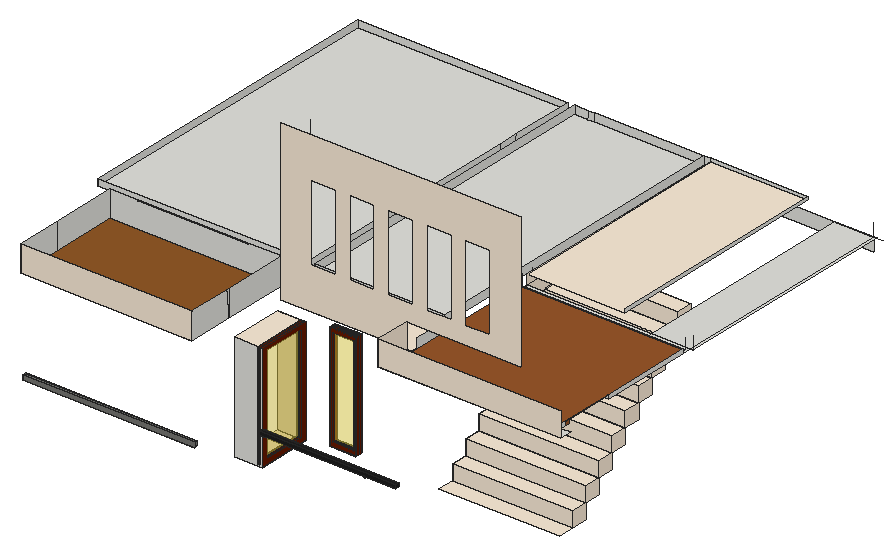
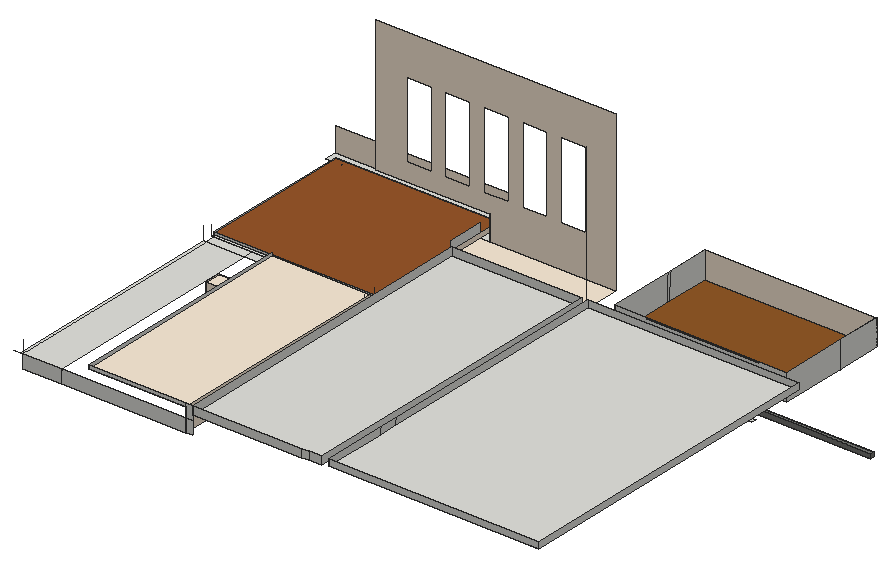
# SketchUp Ruby script. Lengths in inches.
U = 1.inch
M = Sketchup.active_model
def pt(a) = Geom::Point3d.new(a.map { |v| v * U })
def face(e, loops, mat)
  f = e.add_face(loops[0].map { |a| pt(a) })
  loops[1..].each { |l| e.add_face(l.map { |a| pt(a) }).erase! }
  f.material = f.back_material = mat if mat
  f
end
# faces: each face lists its corners as indices into pts; further lists are holes
def faces(e, pts, list, mat = nil) = list.each { |f| face(e, (f[0].is_a?(Array) ? f : [f]).map { |l| l.map { |i| pts[i] } }, mat) }
# xy, xz, yz: faces in a plane at the given z, y or x. An outline is a flat list of corners, or four numbers for a rectangle; further outlines are holes
def ring(l) = l.size == 4 ? [[l[0], l[1]], [l[2], l[1]], [l[2], l[3]], [l[0], l[3]]] : l.each_slice(2).to_a
def flat(e, list, mat, &to3) = list.each { |f| face(e, (f[0].is_a?(Array) ? f : [f]).map { |l| ring(l).map { |u, v| to3.(u, v) } }, mat) }
def xy(e, z, list, mat = nil) = flat(e, list, mat) { |x, y| [x, y, z] }
def xz(e, y, list, mat = nil) = flat(e, list, mat) { |x, z| [x, y, z] }
def yz(e, x, list, mat = nil) = flat(e, list, mat) { |y, z| [x, y, z] }
def lines(e, pts, list) = list.each { |a, b| e.add_line(pt(pts[a]), pt(pts[b])) }
# prism: a flat outline (further loops are holes) pulled along v
def prism(e, loops, v, mat = nil)
  f = face(e, loops, mat); d = Geom::Vector3d.new(v.map { |x| x * U })
  f.pushpull(f.normal.samedirection?(d) ? d.length : -d.length)
end
def box(e, o, s, mat = nil) = prism(e, [[o, [o[0] + s[0], o[1], o[2]], [o[0] + s[0], o[1] + s[1], o[2]], [o[0], o[1] + s[1], o[2]]]], [0, 0, s[2]], mat)
def at(x, y, z, deg = 0) = Geom::Transformation.translation(pt([x, y, z])) * Geom::Transformation.rotation(ORIGIN, Z_AXIS, deg.degrees)
def axes(o, x, y, z) = Geom::Transformation.new([*x, 0, *y, 0, *z, 0, *pt(o).to_a, 1])
def part(name) = M.definitions.add(name)
# library, detail: a bought-in or finely detailed component or shape, given as its bounding box
def library(name, o, s) = part(name).tap { |d| box(d.entities, o, s) }
def detail(e, o, s) = box(e.add_group.entities, o, s)
def put(e, d, t, mat = nil) = e.add_instance(d, t).tap { |i| i.material = mat if mat }
def group(e, t, mat = nil) = e.add_group.tap { |g| g.transformation = t; g.material = mat if mat }.entities
root = M.entities
M.materials.add("[0028_AntiqueWhite]").color = [250, 235, 215]
M.materials.add("[Color B08]").color = [102, 25, 0]
M.materials.add("[Color M00]").color = [255, 255, 255]
M.materials.add("[Color M08]").color = [30, 30, 30]
M.materials.add("[Metal Seamed]").color = [118, 119, 115]
M.materials.add("[Translucent Glass Blue]").color = [255, 231, 67]
M.materials["[Translucent Glass Blue]"].alpha = 0.5
M.materials.add("[Wood Cherry Original]").color = [152, 86, 42]
M.materials.add("[Wood Floor Parquet]").color = [145, 89, 39]
c1 = part("Group\#3")
xy(c1.entities,0,[[0,0,22,2.875],[0,2.875,22,5.5]],"[Color B08]")
xy(c1.entities,2.22,[[2.22,0,19.78,2.875],[2.22,2.875,19.78,5.5]],"[Color B08]")
xy(c1.entities,55.28,[[2.22,0,19.78,2.875],[2.22,2.875,19.78,5.5]],"[Color B08]")
xy(c1.entities,57.5,[[0,0,22,2.875],[0,2.875,22,5.5]],"[Color B08]")
xz(c1.entities,0,[[[0,0,22,57.5],[2.22,2.22,19.78,55.28]]],"[Color B08]")
xz(c1.entities,2.875,[[[0,0,22,57.5],[2.22,2.22,19.78,55.28]]],"[Color B08]")
xz(c1.entities,2.875,[[2.22,2.22,19.78,55.28]],"[Translucent Glass Blue]")
xz(c1.entities,5.5,[[[0,0,22,57.5],[2.22,2.22,19.78,55.28]]],"[Color B08]")
yz(c1.entities,0,[[0,0,2.875,57.5],[2.875,0,5.5,57.5]],"[Color B08]")
yz(c1.entities,2.22,[[0,2.22,2.875,55.28],[2.875,2.22,5.5,55.28]],"[Color B08]")
yz(c1.entities,19.78,[[0,2.22,2.875,55.28],[2.875,2.22,5.5,55.28]],"[Color B08]")
yz(c1.entities,22,[[0,0,2.875,57.5],[2.875,0,5.5,57.5]],"[Color B08]")
c2 = part("Group\#8")
box(c2.entities,[0,0,0],[51.12,12,8])
xy(root,181.1,[[206.5625,238.8,232.3125,288.24]],"[0028_AntiqueWhite]")
xy(root,181.75,[[249.93,292.4375,274.3,298.4375]])
xy(root,187.49,[[355.75,284.99,465.14,299.89]],"[0028_AntiqueWhite]")
xy(root,208.625,[[173.42,194.68,173.5625,194.68,173.71,194.72,173.83,194.79,173.9375,194.89,174.01,195.02,174.05,195.16,174.05,195.31,174.01,195.45,173.94,195.58,173.83,195.68,173.7,195.75,173.5625,195.79,173.42,195.79,173.27,195.75,173.15,195.68,173.04,195.58,172.97,195.45,172.93,195.31,172.93,195.16,172.97,195.02,173.04,194.89,173.15,194.79,173.28,194.71]],"[Color M08]")
xy(root,208.66,[[[50.75,193.58,206.5625,196.4375],[54.79,194.68,54.9375,194.68,55.08,194.72,55.21,194.79,55.3125,194.89,55.38,195.02,55.42,195.16,55.42,195.31,55.38,195.45,55.31,195.58,55.21,195.68,55.08,195.75,54.9375,195.79,54.79,195.79,54.65,195.75,54.52,195.68,54.42,195.58,54.34,195.45,54.31,195.31,54.31,195.16,54.35,195.02,54.42,194.89,54.52,194.79,54.65,194.71],[59.35,194.68,59.5,194.68,59.64,194.72,59.77,194.79,59.875,194.89,59.95,195.02,59.99,195.16,59.98,195.31,59.95,195.45,59.87,195.58,59.77,195.68,59.64,195.75,59.5,195.79,59.35,195.79,59.21,195.75,59.08,195.68,58.98,195.58,58.91,195.45,58.87,195.31,58.87,195.16,58.91,195.02,58.98,194.89,59.09,194.79,59.21,194.71],[63.92,194.68,64.0625,194.68,64.21,194.72,64.33,194.79,64.4375,194.89,64.51,195.02,64.55,195.16,64.55,195.31,64.51,195.45,64.44,195.58,64.33,195.68,64.2,195.75,64.0625,195.79,63.92,195.79,63.77,195.75,63.65,195.68,63.54,195.58,63.47,195.45,63.43,195.31,63.43,195.16,63.47,195.02,63.54,194.89,63.65,194.79,63.78,194.71],[68.48,194.68,68.625,194.68,68.77,194.72,68.9,194.79,69,194.89,69.07,195.02,69.11,195.16,69.11,195.31,69.07,195.45,69,195.58,68.89,195.68,68.77,195.75,68.625,195.79,68.48,195.79,68.34,195.75,68.21,195.68,68.11,195.58,68.03,195.45,67.99,195.31,67.99,195.16,68.03,195.02,68.11,194.89,68.21,194.79,68.34,194.71],[73.04,194.68,73.1875,194.68,73.33,194.72,73.46,194.79,73.5625,194.89,73.63,195.02,73.67,195.16,73.67,195.31,73.63,195.45,73.56,195.58,73.46,195.68,73.33,195.75,73.1875,195.79,73.04,195.79,72.9,195.75,72.77,195.68,72.67,195.58,72.59,195.45,72.56,195.31,72.56,195.16,72.6,195.02,72.67,194.89,72.77,194.79,72.9,194.71],[77.6,194.68,77.75,194.68,77.89,194.72,78.02,194.79,78.125,194.89,78.2,195.02,78.24,195.16,78.23,195.31,78.2,195.45,78.12,195.58,78.02,195.68,77.89,195.75,77.75,195.79,77.6,195.79,77.46,195.75,77.33,195.68,77.23,195.58,77.16,195.45,77.12,195.31,77.12,195.16,77.16,195.02,77.23,194.89,77.34,194.79,77.46,194.71],[82.17,194.68,82.3125,194.68,82.46,194.72,82.58,194.79,82.6875,194.89,82.76,195.02,82.8,195.16,82.8,195.31,82.76,195.45,82.69,195.58,82.58,195.68,82.45,195.75,82.3125,195.79,82.17,195.79,82.02,195.75,81.9,195.68,81.79,195.58,81.72,195.45,81.68,195.31,81.68,195.16,81.72,195.02,81.79,194.89,81.9,194.79,82.03,194.71],[86.73,194.68,86.875,194.68,87.02,194.72,87.15,194.79,87.25,194.89,87.32,195.02,87.36,195.16,87.36,195.31,87.32,195.45,87.25,195.58,87.14,195.68,87.02,195.75,86.875,195.79,86.73,195.79,86.59,195.75,86.46,195.68,86.36,195.58,86.28,195.45,86.24,195.31,86.24,195.16,86.28,195.02,86.36,194.89,86.46,194.79,86.59,194.71],[91.29,194.68,91.4375,194.68,91.58,194.72,91.71,194.79,91.8125,194.89,91.88,195.02,91.92,195.16,91.92,195.31,91.88,195.45,91.81,195.58,91.71,195.68,91.58,195.75,91.4375,195.79,91.29,195.79,91.15,195.75,91.02,195.68,90.92,195.58,90.84,195.45,90.81,195.31,90.81,195.16,90.85,195.02,90.92,194.89,91.02,194.79,91.15,194.71],[95.85,194.68,96,194.68,96.14,194.72,96.27,194.79,96.375,194.89,96.45,195.02,96.49,195.16,96.48,195.31,96.45,195.45,96.37,195.58,96.27,195.68,96.14,195.75,96,195.79,95.85,195.79,95.71,195.75,95.58,195.68,95.48,195.58,95.41,195.45,95.37,195.31,95.37,195.16,95.41,195.02,95.48,194.89,95.59,194.79,95.71,194.71],[104.98,194.68,105.125,194.68,105.27,194.72,105.4,194.79,105.5,194.89,105.57,195.02,105.61,195.16,105.61,195.31,105.57,195.45,105.5,195.58,105.39,195.68,105.27,195.75,105.125,195.79,104.98,195.79,104.84,195.75,104.71,195.68,104.61,195.58,104.53,195.45,104.49,195.31,104.49,195.16,104.53,195.02,104.61,194.89,104.71,194.79,104.84,194.71],[109.54,194.68,109.6875,194.68,109.83,194.72,109.96,194.79,110.0625,194.89,110.13,195.02,110.17,195.16,110.17,195.31,110.13,195.45,110.06,195.58,109.96,195.68,109.83,195.75,109.6875,195.79,109.54,195.79,109.4,195.75,109.27,195.68,109.17,195.58,109.09,195.45,109.06,195.31,109.06,195.16,109.1,195.02,109.17,194.89,109.27,194.79,109.4,194.71],[114.1,194.68,114.25,194.68,114.39,194.72,114.52,194.79,114.625,194.89,114.7,195.02,114.74,195.16,114.73,195.31,114.7,195.45,114.62,195.58,114.52,195.68,114.39,195.75,114.25,195.79,114.1,195.79,113.96,195.75,113.83,195.68,113.73,195.58,113.66,195.45,113.62,195.31,113.62,195.16,113.66,195.02,113.73,194.89,113.84,194.79,113.96,194.71],[118.67,194.68,118.8125,194.68,118.96,194.72,119.08,194.79,119.1875,194.89,119.26,195.02,119.3,195.16,119.3,195.31,119.26,195.45,119.19,195.58,119.08,195.68,118.95,195.75,118.8125,195.79,118.67,195.79,118.52,195.75,118.4,195.68,118.29,195.58,118.22,195.45,118.18,195.31,118.18,195.16,118.22,195.02,118.29,194.89,118.4,194.79,118.53,194.71],[123.23,194.68,123.375,194.68,123.52,194.72,123.65,194.79,123.75,194.89,123.82,195.02,123.86,195.16,123.86,195.31,123.82,195.45,123.75,195.58,123.64,195.68,123.52,195.75,123.375,195.79,123.23,195.79,123.09,195.75,122.96,195.68,122.86,195.58,122.78,195.45,122.74,195.31,122.74,195.16,122.78,195.02,122.86,194.89,122.96,194.79,123.09,194.71],[127.79,194.68,127.9375,194.68,128.08,194.72,128.21,194.79,128.3125,194.89,128.38,195.02,128.42,195.16,128.42,195.31,128.38,195.45,128.31,195.58,128.21,195.68,128.08,195.75,127.9375,195.79,127.79,195.79,127.65,195.75,127.52,195.68,127.42,195.58,127.34,195.45,127.31,195.31,127.31,195.16,127.35,195.02,127.42,194.89,127.52,194.79,127.65,194.71],[132.35,194.68,132.5,194.68,132.64,194.72,132.77,194.79,132.875,194.89,132.95,195.02,132.99,195.16,132.98,195.31,132.95,195.45,132.87,195.58,132.77,195.68,132.64,195.75,132.5,195.79,132.35,195.79,132.21,195.75,132.08,195.68,131.98,195.58,131.91,195.45,131.87,195.31,131.87,195.16,131.91,195.02,131.98,194.89,132.09,194.79,132.21,194.71],[136.92,194.68,137.0625,194.68,137.21,194.72,137.33,194.79,137.4375,194.89,137.51,195.02,137.55,195.16,137.55,195.31,137.51,195.45,137.44,195.58,137.33,195.68,137.2,195.75,137.0625,195.79,136.92,195.79,136.77,195.75,136.65,195.68,136.54,195.58,136.47,195.45,136.43,195.31,136.43,195.16,136.47,195.02,136.54,194.89,136.65,194.79,136.78,194.71],[141.48,194.68,141.625,194.68,141.77,194.72,141.9,194.79,142,194.89,142.07,195.02,142.11,195.16,142.11,195.31,142.07,195.45,142,195.58,141.89,195.68,141.77,195.75,141.625,195.79,141.48,195.79,141.34,195.75,141.21,195.68,141.11,195.58,141.03,195.45,140.99,195.31,140.99,195.16,141.03,195.02,141.11,194.89,141.21,194.79,141.34,194.71],[146.04,194.68,146.1875,194.68,146.33,194.72,146.46,194.79,146.5625,194.89,146.63,195.02,146.67,195.16,146.67,195.31,146.63,195.45,146.56,195.58,146.46,195.68,146.33,195.75,146.1875,195.79,146.04,195.79,145.9,195.75,145.77,195.68,145.67,195.58,145.59,195.45,145.56,195.31,145.56,195.16,145.6,195.02,145.67,194.89,145.77,194.79,145.9,194.71],[150.6,194.68,150.75,194.68,150.89,194.72,151.02,194.79,151.125,194.89,151.2,195.02,151.24,195.16,151.23,195.31,151.2,195.45,151.12,195.58,151.02,195.68,150.89,195.75,150.75,195.79,150.6,195.79,150.46,195.75,150.33,195.68,150.23,195.58,150.16,195.45,150.12,195.31,150.12,195.16,150.16,195.02,150.23,194.89,150.34,194.79,150.46,194.71],[155.17,194.68,155.3125,194.68,155.46,194.72,155.58,194.79,155.6875,194.89,155.76,195.02,155.8,195.16,155.8,195.31,155.76,195.45,155.69,195.58,155.58,195.68,155.45,195.75,155.3125,195.79,155.17,195.79,155.02,195.75,154.9,195.68,154.79,195.58,154.72,195.45,154.68,195.31,154.68,195.16,154.72,195.02,154.79,194.89,154.9,194.79,155.03,194.71],[159.73,194.68,159.875,194.68,160.02,194.72,160.15,194.79,160.25,194.89,160.32,195.02,160.36,195.16,160.36,195.31,160.32,195.45,160.25,195.58,160.14,195.68,160.02,195.75,159.875,195.79,159.73,195.79,159.59,195.75,159.46,195.68,159.36,195.58,159.28,195.45,159.24,195.31,159.24,195.16,159.28,195.02,159.36,194.89,159.46,194.79,159.59,194.71],[164.29,194.68,164.4375,194.68,164.58,194.72,164.71,194.79,164.8125,194.89,164.88,195.02,164.92,195.16,164.92,195.31,164.88,195.45,164.81,195.58,164.71,195.68,164.58,195.75,164.4375,195.79,164.29,195.79,164.15,195.75,164.02,195.68,163.92,195.58,163.84,195.45,163.81,195.31,163.81,195.16,163.85,195.02,163.92,194.89,164.02,194.79,164.15,194.71],[168.85,194.68,169,194.68,169.14,194.72,169.27,194.79,169.375,194.89,169.45,195.02,169.49,195.16,169.48,195.31,169.45,195.45,169.37,195.58,169.27,195.68,169.14,195.75,169,195.79,168.85,195.79,168.71,195.75,168.58,195.68,168.48,195.58,168.41,195.45,168.37,195.31,168.37,195.16,168.41,195.02,168.48,194.89,168.59,194.79,168.71,194.71],[177.98,194.68,178.125,194.68,178.27,194.72,178.4,194.79,178.5,194.89,178.57,195.02,178.61,195.16,178.61,195.31,178.57,195.45,178.5,195.58,178.39,195.68,178.27,195.75,178.125,195.79,177.98,195.79,177.84,195.75,177.71,195.68,177.61,195.58,177.53,195.45,177.49,195.31,177.49,195.16,177.53,195.02,177.61,194.89,177.71,194.79,177.84,194.71],[182.54,194.68,182.6875,194.68,182.83,194.72,182.96,194.79,183.0625,194.89,183.13,195.02,183.17,195.16,183.17,195.31,183.13,195.45,183.06,195.58,182.96,195.68,182.83,195.75,182.6875,195.79,182.54,195.79,182.4,195.75,182.27,195.68,182.17,195.58,182.09,195.45,182.06,195.31,182.06,195.16,182.1,195.02,182.17,194.89,182.27,194.79,182.4,194.71],[187.1,194.68,187.25,194.68,187.39,194.72,187.52,194.79,187.625,194.89,187.7,195.02,187.74,195.16,187.73,195.31,187.7,195.45,187.62,195.58,187.52,195.68,187.39,195.75,187.25,195.79,187.1,195.79,186.96,195.75,186.83,195.68,186.73,195.58,186.66,195.45,186.62,195.31,186.62,195.16,186.66,195.02,186.73,194.89,186.84,194.79,186.96,194.71],[191.67,194.68,191.8125,194.68,191.96,194.72,192.08,194.79,192.1875,194.89,192.26,195.02,192.3,195.16,192.3,195.31,192.26,195.45,192.19,195.58,192.08,195.68,191.95,195.75,191.8125,195.79,191.67,195.79,191.52,195.75,191.4,195.68,191.29,195.58,191.22,195.45,191.18,195.31,191.18,195.16,191.22,195.02,191.29,194.89,191.4,194.79,191.53,194.71],[196.23,194.68,196.375,194.68,196.52,194.72,196.65,194.79,196.75,194.89,196.82,195.02,196.86,195.16,196.86,195.31,196.82,195.45,196.75,195.58,196.64,195.68,196.52,195.75,196.375,195.79,196.23,195.79,196.09,195.75,195.96,195.68,195.86,195.58,195.78,195.45,195.74,195.31,195.74,195.16,195.78,195.02,195.86,194.89,195.96,194.79,196.09,194.71],[200.79,194.68,200.9375,194.68,201.08,194.72,201.21,194.79,201.3125,194.89,201.38,195.02,201.42,195.16,201.42,195.31,201.38,195.45,201.31,195.58,201.21,195.68,201.08,195.75,200.9375,195.79,200.79,195.79,200.65,195.75,200.52,195.68,200.42,195.58,200.34,195.45,200.31,195.31,200.31,195.16,200.35,195.02,200.42,194.89,200.52,194.79,200.65,194.71],[100.42,194.68,100.5625,194.68,100.71,194.72,100.83,194.79,100.9375,194.89,101.01,195.02,101.05,195.16,101.05,195.31,101.01,195.45,100.94,195.58,100.83,195.68,100.7,195.75,100.5625,195.79,100.42,195.79,100.27,195.75,100.15,195.68,100.04,195.58,99.97,195.45,99.93,195.31,99.93,195.16,99.97,195.02,100.04,194.89,100.15,194.79,100.28,194.71]]],"[Metal Seamed]")
xy(root,208.9375,[[205.35,194.68,205.5,194.68,205.64,194.72,205.77,194.79,205.875,194.89,205.95,195.02,205.99,195.16,205.98,195.31,205.95,195.45,205.87,195.58,205.77,195.68,205.64,195.75,205.5,195.79,205.35,195.79,205.21,195.75,205.08,195.68,204.98,195.58,204.91,195.45,204.87,195.31,204.87,195.16,204.91,195.02,204.98,194.89,205.09,194.79,205.21,194.71]],"[Color M08]")
xy(root,209.625,[[353.9,235.17,354.0625,235.2,354.21,235.26,354.34,235.36,354.44,235.49,354.5,235.64,354.53,235.8,354.5,235.96,354.44,236.11,354.34,236.24,354.21,236.34,354.0625,236.4,353.9,236.42,353.74,236.4,353.59,236.34,353.46,236.24,353.36,236.11,353.3,235.96,353.28,235.8,353.3,235.64,353.36,235.49,353.46,235.36,353.59,235.26,353.74,235.2]],"[Color M08]")
xy(root,209.97,[[[232.3125,234.5,232.3125,238.33,288.38,238.33,288.23,238.14,288.1,237.84,288.0625,237.51,288.1,237.19,288.23,236.89,288.43,236.63,288.6875,236.43,288.99,236.31,289.3125,236.26,289.64,236.31,289.9375,236.43,290.2,236.63,290.39,236.89,290.52,237.19,290.5625,237.51,290.52,237.84,290.39,238.14,290.25,238.33,302.34,238.33,302.19,238.14,302.07,237.84,302.03,237.51,302.07,237.19,302.19,236.89,302.39,236.63,302.65,236.43,302.95,236.31,303.28,236.26,303.6,236.31,303.9,236.43,304.16,236.63,304.36,236.89,304.48,237.19,304.53,237.51,304.48,237.84,304.36,238.14,304.21,238.33,356.53,238.33,356.53,234.5,330.39,234.5,330.4,234.53,330.35,234.86,330.23,235.16,330.03,235.42,329.77,235.62,329.47,235.74,329.15,235.78,328.82,235.74,328.52,235.62,328.26,235.42,328.0625,235.16,327.9375,234.86,327.9,234.53,327.9,234.5],[316.02,235.77,316.35,235.82,316.65,235.94,316.91,236.14,317.11,236.4,317.23,236.7,317.27,237.02,317.23,237.35,317.11,237.65,316.91,237.91,316.65,238.11,316.35,238.23,316.02,238.27,315.7,238.23,315.4,238.11,315.14,237.91,314.94,237.65,314.82,237.35,314.77,237.02,314.82,236.7,314.94,236.4,315.14,236.14,315.4,235.94,315.7,235.82],[341.03,235.41,341.36,235.45,341.66,235.58,341.92,235.77,342.12,236.03,342.24,236.34,342.28,236.66,342.24,236.98,342.12,237.28,341.92,237.54,341.66,237.74,341.36,237.87,341.03,237.91,340.71,237.87,340.41,237.74,340.15,237.54,339.95,237.28,339.83,236.98,339.78,236.66,339.83,236.34,339.95,236.03,340.15,235.77,340.41,235.58,340.71,235.45],[276.2,235.93,276.375,235.96,276.54,236.03,276.68,236.14,276.79,236.29,276.85,236.45,276.87,236.63,276.84,236.81,276.77,236.97,276.66,237.11,276.52,237.22,276.35,237.29,276.17,237.31,275.99,237.28,275.83,237.21,275.6875,237.09,275.58,236.95,275.52,236.78,275.5,236.61,275.52,236.43,275.59,236.26,275.71,236.12,275.85,236.02,276.02,235.95],[269.26,235.93,269.4375,235.96,269.6,236.03,269.74,236.14,269.85,236.29,269.91,236.45,269.93,236.63,269.91,236.81,269.83,236.97,269.72,237.11,269.58,237.22,269.41,237.29,269.23,237.31,269.06,237.28,268.89,237.21,268.75,237.09,268.64,236.95,268.58,236.78,268.56,236.61,268.59,236.43,268.66,236.26,268.77,236.12,268.91,236.02,269.08,235.95],[263.76,235.93,263.9375,235.96,264.1,236.03,264.24,236.14,264.35,236.29,264.41,236.45,264.43,236.63,264.41,236.81,264.33,236.97,264.22,237.11,264.08,237.22,263.91,237.29,263.73,237.31,263.56,237.28,263.39,237.21,263.25,237.09,263.14,236.95,263.08,236.78,263.06,236.61,263.09,236.43,263.16,236.26,263.27,236.12,263.41,236.02,263.58,235.95],[258.32,235.93,258.5,235.96,258.66,236.03,258.8,236.14,258.91,236.29,258.98,236.45,259,236.63,258.97,236.81,258.9,236.97,258.79,237.11,258.64,237.22,258.47,237.29,258.3,237.31,258.12,237.28,257.95,237.21,257.8125,237.09,257.71,236.95,257.64,236.78,257.62,236.61,257.65,236.43,257.72,236.26,257.83,236.12,257.98,236.02,258.14,235.95],[252.88,235.93,253.0625,235.96,253.23,236.03,253.37,236.14,253.47,236.29,253.54,236.45,253.56,236.63,253.53,236.81,253.46,236.97,253.35,237.11,253.2,237.22,253.04,237.29,252.86,237.31,252.68,237.28,252.52,237.21,252.375,237.09,252.27,236.95,252.2,236.78,252.18,236.61,252.21,236.43,252.28,236.26,252.39,236.12,252.54,236.02,252.71,235.95],[247.45,235.93,247.625,235.96,247.79,236.03,247.93,236.14,248.04,236.29,248.1,236.45,248.12,236.63,248.09,236.81,248.02,236.97,247.91,237.11,247.77,237.22,247.6,237.29,247.42,237.31,247.24,237.28,247.08,237.21,246.9375,237.09,246.83,236.95,246.77,236.78,246.75,236.61,246.77,236.43,246.84,236.26,246.96,236.12,247.1,236.02,247.27,235.95],[242.01,235.93,242.1875,235.96,242.35,236.03,242.49,236.14,242.6,236.29,242.66,236.45,242.68,236.63,242.66,236.81,242.58,236.97,242.47,237.11,242.33,237.22,242.16,237.29,241.98,237.31,241.81,237.28,241.64,237.21,241.5,237.09,241.39,236.95,241.33,236.78,241.31,236.61,241.34,236.43,241.41,236.26,241.52,236.12,241.66,236.02,241.83,235.95],[236.57,235.93,236.75,235.96,236.91,236.03,237.05,236.14,237.16,236.29,237.23,236.45,237.25,236.63,237.22,236.81,237.15,236.97,237.04,237.11,236.89,237.22,236.72,237.29,236.55,237.31,236.37,237.28,236.2,237.21,236.0625,237.09,235.96,236.95,235.89,236.78,235.87,236.61,235.9,236.43,235.97,236.26,236.08,236.12,236.23,236.02,236.39,235.95]],[289.3125,236.26,288.99,236.31,288.6875,236.43,288.43,236.63,288.23,236.89,288.1,237.19,288.0625,237.51,288.1,237.84,288.23,238.14,288.38,238.33,290.25,238.33,290.39,238.14,290.52,237.84,290.5625,237.51,290.52,237.19,290.39,236.89,290.2,236.63,289.9375,236.43,289.64,236.31],[303.28,236.26,302.95,236.31,302.65,236.43,302.39,236.63,302.19,236.89,302.07,237.19,302.03,237.51,302.07,237.84,302.19,238.14,302.34,238.33,304.21,238.33,304.36,238.14,304.48,237.84,304.53,237.51,304.48,237.19,304.36,236.89,304.16,236.63,303.9,236.43,303.6,236.31]],"[Color M00]")
xy(root,209.97,[[329.15,233.28,329.47,233.33,329.77,233.45,330.03,233.65,330.23,233.91,330.35,234.21,330.39,234.5,327.9,234.5,327.9375,234.21,328.0625,233.91,328.26,233.65,328.52,233.45,328.82,233.33],[327.9,234.5,330.39,234.5,330.4,234.53,330.35,234.86,330.23,235.16,330.03,235.42,329.77,235.62,329.47,235.74,329.15,235.78,328.82,235.74,328.52,235.62,328.26,235.42,328.0625,235.16,327.9375,234.86,327.9,234.53],[288.38,238.33,290.25,238.33,290.2,238.4,289.9375,238.6,289.64,238.72,289.3125,238.76,288.99,238.72,288.6875,238.6,288.43,238.4],[302.34,238.33,304.21,238.33,304.16,238.4,303.9,238.6,303.6,238.72,303.28,238.76,302.95,238.72,302.65,238.6,302.39,238.4]],"[Color M08]")
xy(root,213,[[232.3125,234.5,356.53,238.33]],"[Color M08]")
xy(root,213,[[50.75,193.51,206.5625,196.4375]],"[Metal Seamed]")
xy(root,272.875,[[174.56,292.48,78.68,292.59,78.6875,296.84,174.5625,296.73]])
xy(root,278.41,[[206.5625,238.8,232.3125,288.24]],"[0028_AntiqueWhite]")
xy(root,278.54,[[249.93,292.4375,274.3,298.4375]])
xy(root,297,[[50.7,190.5,50.75,231.9375,50.75,190.5]])
xy(root,297,[[206.51,190.32,50.75,190.5,50.75,231.9375,50.68,231.9375,50.75,292.625,206.5625,292.44,206.63,292.44,206.5625,231.9375]],"[Wood Floor Parquet]")
xy(root,309,[[346.5625,227.125,346.5625,259.125,355.625,259.125,355.625,238.03,503.75,238.03,503.75,238.0625,512.4375,238.0625,512.4375,227.125],[468.75,292.4375,503.75,376.0625],[355.625,376.0625,468.75,384.87],[468.75,376.0625,503.75,384.87],[468.75,384.87,503.75,592.9375],
  [503.75,384.87,506.4375,592.9375]])
xy(root,309,[[232.3125,259.125,355.625,292.4375]],"[0028_AntiqueWhite]")
xy(root,311.0625,[[355.625,376.0625,503.75,379.25]])
xy(root,312.375,[[468.75,246.875,503.75,292.4375]])
xy(root,312.375,[[471.79,242.8125,476.92,246.875],[480.23,242.8125,485.67,246.875],[489.36,242.8125,494.11,246.875],[497.73,242.8125,503.75,246.875]],"[Wood Cherry Original]")
xy(root,312.75,[[355.625,238.03,503.75,376.0625]],"[Wood Cherry Original]")
xy(root,313.625,[[232.3125,298.4375,349.625,592.9375]])
xy(root,315,[[35.1875,298.4375,226.3125,592.9375]])
xy(root,318.0625,[[355.625,384.87,444.4375,592.9375]],"[0028_AntiqueWhite]")
xz(root,190.5,[[50.7,297,50.75,321],[50.7,297,50.75,321]])
xz(root,196.4375,[[50.75,208.66,206.5625,213]],"[Metal Seamed]")
xz(root,227.125,[[346.5625,309,512.4375,331.3125]],"[0028_AntiqueWhite]")
xz(root,231.9375,[[50.68,297,50.75,321]])
xz(root,234.5,[[232.3125,209.97,356.53,213]],"[Color M08]")
xz(root,238.03,[[355.625,309,503.75,312.75]])
xz(root,238.33,[[232.3125,209.97,356.53,213]],"[Color M08]")
xz(root,238.8,[[206.5625,181.1,232.3125,278.41]])
xz(root,259.125,[[[232.3125,309,346.5625,309,346.5625,331.3125,450.25,331.3125,450.25,453,232.3125,453],[259.68,347.02,282.31,416.46],[294.75,347.02,317.37,416.46],[329.81,347.02,352.43,416.46],[364.87,347.02,387.5,416.46],[399.93,347.02,422.56,416.46]]],"[0028_AntiqueWhite]")
xz(root,288.24,[[206.5625,181.1,232.3125,278.41]],"[0028_AntiqueWhite]")
xz(root,292.4375,[[468.75,309,503.75,312.375]])
xz(root,292.44,[[206.5625,297,206.63,321]])
xz(root,298.4375,[[232.3125,313.625,349.625,321],[35.1875,315,226.3125,321]])
xz(root,376.0625,[[355.625,309,503.75,311.0625],[355.625,311.0625,503.75,312.75]])
xz(root,592.9375,[[349.625,297,355.625,309],[355.625,297,468.75,309],[468.75,297,503.75,309],[349.625,309,355.625,321],[232.3125,313.625,244.68,321],
  [244.68,313.625,250.68,321],[250.68,313.625,349.625,321],[35.1875,315,226.3125,321],[355.625,318.0625,444.4375,321]])
yz(root,35.1875,[[298.4375,315,592.9375,321]])
yz(root,50.75,[[190.5,297,231.9375,321]])
yz(root,50.75,[[193.58,208.66,193.51,213,196.4375,213,196.4375,208.66]],"[Metal Seamed]")
yz(root,206.5625,[[190.5,297,231.9375,321]])
yz(root,226.3125,[[298.4375,315,516.13,321],[516.13,315,534.07,321],[534.07,315,592.9375,321]])
yz(root,232.3125,[[298.4375,313.625,592.9375,321]])
yz(root,232.3125,[[234.5,209.97,238.33,213]],"[Color M08]")
yz(root,249.93,[[292.4375,181.75,298.4375,278.54]])
yz(root,274.3,[[292.4375,181.75,298.4375,278.54]])
yz(root,346.5625,[[227.125,309,259.125,331.3125]],"[0028_AntiqueWhite]")
yz(root,349.625,[[298.4375,313.625,592.9375,321]])
yz(root,355.625,[[259.125,312.75,292.4375,321]])
yz(root,355.625,[[375.81,297,592.9375,297,592.9375,309,376.0625,309,376.0625,312.75,375.81,312.75],[238.03,309,292.4375,312.75],[384.87,309,592.9375,318.0625]],"[0028_AntiqueWhite]")
yz(root,356.53,[[234.5,209.97,238.33,213]],"[Color M08]")
yz(root,444.4375,[[384.87,318.0625,592.9375,321]])
yz(root,503.75,[[238.03,309,238.03,312.75,292.4375,312.75,292.4375,312.375,242.8125,312.375,242.8125,309],[292.4375,309,376.0625,312.75]])
yz(root,503.75,[[242.8125,309,246.875,312.375]],"[Wood Cherry Original]")
p = [[50.75,193.51,213],[50.75,193.58,208.66],[206.5625,193.58,208.66],[206.5625,193.51,213],[206.51,190.32,321],[50.75,190.5,321],
  [50.75,190.5,297],[206.51,190.32,297],[206.5625,231.9375,297],[206.5625,231.9375,321],[206.52,193.51,321],[50.75,231.9375,321],
  [50.75,231.9375,297],[50.7,190.5,297],[50.7,190.5,321],[50.75,292.625,321],[50.75,292.625,297],[50.68,231.9375,297],
  [50.68,231.9375,321],[206.63,292.44,297],[206.63,292.44,321],[76.05,292.6,321],[76.05,292.6,320.1875],[177.59,292.48,320.1875],
  [177.59,292.48,321],[206.5625,292.44,321],[206.5625,292.44,297],[232.3125,292.4375,309],[232.3125,292.4375,441],[506.4375,384.87,321],
  [506.4375,384.87,309],[503.75,592.9375,309],[503.75,592.9375,321],[512.4375,592.9375,309],[506.4375,592.9375,309],[355.625,379.25,311.0625],
  [355.625,379.25,321],[503.75,379.25,311.0625],[503.75,379.25,321],[355.625,390.49,321],[355.625,390.49,318.0625]]
faces(root,p,[[0,1,2,3]],"[Metal Seamed]")
faces(root,p,[[4,5,6,7]],"[0028_AntiqueWhite]")
faces(root,p,[[8,9,10,4,7],[11,12,13,14],[15,16,17,18],[19,20,9,8],[15,21,22,23,24,25,26,16],[22,23,24,21]])
lines(root,p,[[27,28],[29,30],[31,32],[33,34],[35,36],[37,38],[39,40]])
put(root,c1,axes([250.11,292.95,181.75],[1.09986,0,0],[0,0.7565,0],[0,0,1.68331]))
put(root,c1,axes([232.3125,238.8,182.42],[0,2.24716,0],[-0.85,0,0],[0,0,1.66944]))
put(root,c2,axes([355.75,299.89,187.49],[2.14,0,0],[0,1.24129,0],[0,0,1.71626]),"[0028_AntiqueWhite]")
put(root,c2,axes([355.75,314.78,201.22],[2.14,0,0],[0,1.24129,0],[0,0,1.71626]),"[0028_AntiqueWhite]")
put(root,c2,axes([355.75,329.68,214.95],[2.14,0,0],[0,1.24129,0],[0,0,1.71626]),"[0028_AntiqueWhite]")
put(root,c2,axes([355.75,344.57,228.68],[2.14,0,0],[0,1.24129,0],[0,0,1.71626]),"[0028_AntiqueWhite]")
put(root,c2,axes([355.75,359.47,242.41],[2.14,0,0],[0,1.24129,0],[0,0,1.71626]),"[0028_AntiqueWhite]")
put(root,c2,axes([355.75,374.36,256.14],[2.14,0,0],[0,1.24129,0],[0,0,1.71626]),"[0028_AntiqueWhite]")
put(root,c2,axes([355.75,389.26,269.87],[2.14,0,0],[0,1.24129,0],[0,0,1.71626]),"[0028_AntiqueWhite]")
put(root,c2,axes([355.75,404.15,283.6],[2.14,0,0],[0,1.24129,0],[0,0,1.71626]),"[0028_AntiqueWhite]")
put(root,c2,axes([355.75,419.05,297.33],[2.14,0,0],[0,1.24129,0],[0,0,1.71626]),"[0028_AntiqueWhite]")
